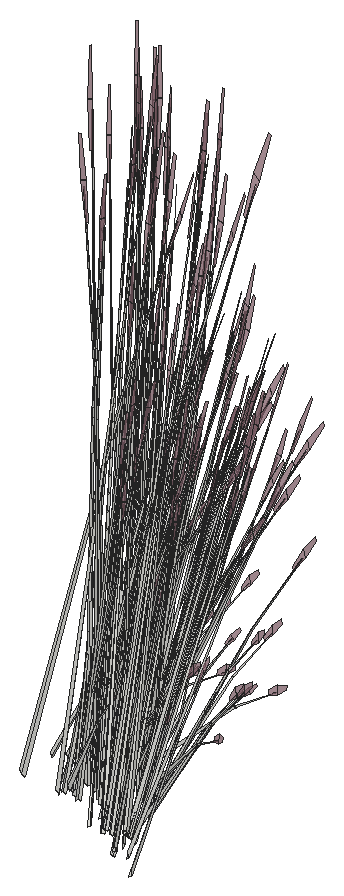
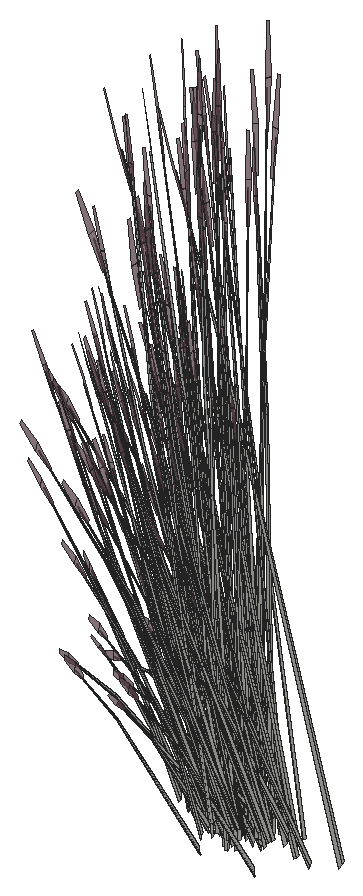
# SketchUp Ruby script. Lengths in inches.
U = 1.inch
M = Sketchup.active_model
def pt(a) = Geom::Point3d.new(a.map { |v| v * U })
def face(e, loops, mat)
  f = e.add_face(loops[0].map { |a| pt(a) })
  loops[1..].each { |l| e.add_face(l.map { |a| pt(a) }).erase! }
  f.material = f.back_material = mat if mat
  f
end
# faces: each face lists its corners as indices into pts; further lists are holes
def faces(e, pts, list, mat = nil) = list.each { |f| face(e, (f[0].is_a?(Array) ? f : [f]).map { |l| l.map { |i| pts[i] } }, mat) }
# xy, xz, yz: faces in a plane at the given z, y or x. An outline is a flat list of corners, or four numbers for a rectangle; further outlines are holes
def ring(l) = l.size == 4 ? [[l[0], l[1]], [l[2], l[1]], [l[2], l[3]], [l[0], l[3]]] : l.each_slice(2).to_a
def flat(e, list, mat, &to3) = list.each { |f| face(e, (f[0].is_a?(Array) ? f : [f]).map { |l| ring(l).map { |u, v| to3.(u, v) } }, mat) }
def xy(e, z, list, mat = nil) = flat(e, list, mat) { |x, y| [x, y, z] }
def xz(e, y, list, mat = nil) = flat(e, list, mat) { |x, z| [x, y, z] }
def yz(e, x, list, mat = nil) = flat(e, list, mat) { |y, z| [x, y, z] }
def lines(e, pts, list) = list.each { |a, b| e.add_line(pt(pts[a]), pt(pts[b])) }
# prism: a flat outline (further loops are holes) pulled along v
def prism(e, loops, v, mat = nil)
  f = face(e, loops, mat); d = Geom::Vector3d.new(v.map { |x| x * U })
  f.pushpull(f.normal.samedirection?(d) ? d.length : -d.length)
end
def box(e, o, s, mat = nil) = prism(e, [[o, [o[0] + s[0], o[1], o[2]], [o[0] + s[0], o[1] + s[1], o[2]], [o[0], o[1] + s[1], o[2]]]], [0, 0, s[2]], mat)
def at(x, y, z, deg = 0) = Geom::Transformation.translation(pt([x, y, z])) * Geom::Transformation.rotation(ORIGIN, Z_AXIS, deg.degrees)
def axes(o, x, y, z) = Geom::Transformation.new([*x, 0, *y, 0, *z, 0, *pt(o).to_a, 1])
def part(name) = M.definitions.add(name)
# library, detail: a bought-in or finely detailed component or shape, given as its bounding box
def library(name, o, s) = part(name).tap { |d| box(d.entities, o, s) }
def detail(e, o, s) = box(e.add_group.entities, o, s)
def put(e, d, t, mat = nil) = e.add_instance(d, t).tap { |i| i.material = mat if mat }
def group(e, t, mat = nil) = e.add_group.tap { |g| g.transformation = t; g.material = mat if mat }.entities
root = M.entities
M.materials.add("LightPink_Translucent").color = [144, 107, 117]
M.materials["LightPink_Translucent"].alpha = 0.75
c1 = part("blade")
p = [[2.15,0.21,22],[0,0.17,0],[0.09,0.45,0],[2.18,0.31,22],[2.29,0.31,22],[0.38,0.45,0],
  [2.48,0.24,33],[2.49,0.24,33],[2.48,0.22,33]]
faces(c1.entities,p,[[0,1,2,3],[4,5,2,3],[6,3,4,7],[8,0,3,6]])
c2 = part("seeds")
p = [[0.3,-0.1,1.38],[-0.01,-0.03,1.59],[-0.01,-0.03,0.03],[0.14,-0.07,-0.07],[0.29,-0.03,3],[0.15,0.01,3.11]]
faces(c2.entities,p,[[0,1,2,3],[1,0,4,5]],"LightPink_Translucent")
c3 = part("blade with seeds")
put(c3.entities,c1,at(0,0,0))
put(c3.entities,c2,axes([2.4,0.25,30.99],[1.5799,-0.05474,1.17369],[-0.12525,1.92788,0.29478],[-0.07173,-0.02425,1.56792]))
put(root,c3,axes([679.03,338.02,392.3],[-0.2167,0.29065,0.95334],[-0.18626,-0.3905,0.70045],[0.17898,-0.09785,0.20998]))
put(root,c3,axes([683.1,338.02,392.3],[-0.2167,0.29065,0.95334],[-0.18626,-0.3905,0.70045],[0.17898,-0.09785,0.20998]))
put(root,c3,axes([687.03,333.57,393.93],[-0.47939,0.19405,0.05337],[-0.23464,-0.35385,0.42015],[0.0463,0.15598,0.64067]))
put(root,c3,axes([685.74,333.11,393.76],[-0.4402,0.30062,-0.29394],[-0.41671,-0.34326,0.37948],[-0.0634,0.1744,0.72609]))
put(root,c3,axes([684.22,333.02,393.91],[-0.01617,0.11299,1.45204],[0.45894,0.39307,-0.22964],[-0.12015,0.18588,0.11645]))
put(root,c3,axes([685.69,332.76,394.48],[0.71502,0.02829,-0.11203],[-0.01954,0.53563,-0.62183],[-0.04967,0.20629,0.94486]))
put(root,c3,axes([687.01,333.36,394.18],[0.63664,-0.26583,-0.10093],[0.31286,0.47181,-0.56021],[0.084,0.19882,0.85122]))
put(root,c3,axes([687.2,333.53,394.2],[-0.64106,-0.14927,0.44225],[0.21921,-0.49074,0.36465],[0.03852,0.19299,0.91512]))
put(root,c3,axes([686.02,334.27,392.3],[-0.01684,-0.3395,0.95334],[0.42072,0.24214,0.70045],[-0.08274,0.16182,0.20998]))
put(root,c3,axes([678.72,339.11,393.76],[0.56631,-0.0816,-0.29394],[0.14954,0.46647,0.37948],[0.16229,-0.12529,0.72609]))
put(root,c3,axes([682.79,339.11,393.76],[0.56631,-0.0816,-0.29394],[0.14954,0.46647,0.37948],[0.16229,-0.12529,0.72609]))
put(root,c3,axes([687.13,333.46,391.24],[0.10529,-0.03107,1.46364],[0.63335,0.17101,-0.2236],[0.01852,0.19274,0.24931]))
put(root,c3,axes([679.47,339.53,392.21],[-0.07581,-0.65151,-0.24149],[0.7896,-0.03939,-0.41502],[0.13904,-0.08678,1.32557]))
put(root,c3,axes([686.18,332.96,394.15],[0.46573,0.38364,-0.47077],[-0.49199,0.33598,-0.36465],[-0.07086,0.19492,0.90078]))
put(root,c3,axes([682.33,339.38,394.19],[-0.56631,0.0816,0.29394],[-0.14954,-0.46647,-0.37948],[0.16229,-0.12529,0.72609]))
put(root,c3,axes([685.67,333.54,392.34],[0.59102,-0.10111,0.05401],[0.13587,0.40735,-0.71633],[-0.03747,0.2062,0.64209]))
put(root,c3,axes([687.56,333.34,393.89],[0.63954,0.14313,-0.42412],[-0.21921,0.49074,-0.32852],[0.05864,0.19758,0.81151]))
put(root,c3,axes([687.92,332.32,393.22],[-0.14872,-0.18332,1.42242],[0.6872,-0.15433,0.11501],[0.15531,0.28779,0.60807]))
put(root,c3,axes([679.36,338.09,391.68],[0.60696,0.14127,-0.25712],[-0.15283,0.49751,0.25712],[0.12236,-0.05737,1.15348]))
put(root,c3,axes([687.27,333.64,393.76],[-0.19614,0.43908,-0.29394],[-0.57222,-0.12807,0.37948],[0.05247,0.17678,0.72609]))
put(root,c3,axes([686.03,332.79,394.43],[-0.01693,0.52814,-0.65454],[-0.71285,-0.03547,0.07899],[-0.07523,0.22375,0.92591]))
put(root,c3,axes([684.17,334.18,393.91],[0.07381,-0.03447,1.47228],[0.61004,0.22929,-0.13912],[-0.01434,0.19091,0.26054]))
put(root,c3,axes([678.77,339.31,393.93],[0.44663,0.24013,0.05337],[-0.26003,0.34195,0.42015],[0.14319,-0.11055,0.64067]))
put(root,c3,axes([682.84,339.31,393.93],[0.44663,0.24013,0.05337],[-0.26003,0.34195,0.42015],[0.14319,-0.11055,0.64067]))
put(root,c3,axes([678.65,339.21,393.93],[0.16135,0.52549,0.39842],[-0.63294,0.0912,0.32852],[0.18654,-0.12359,0.82444]))
put(root,c3,axes([682.72,339.21,393.93],[0.16135,0.52549,0.39842],[-0.63294,0.0912,0.32852],[0.18654,-0.12359,0.82444]))
put(root,c3,axes([680.36,339.84,393.91],[0.09028,-0.08697,1.45204],[-0.11555,-0.53348,-0.22964],[0.22652,-0.10115,0.11645]))
put(root,c3,axes([684.42,339.84,393.91],[0.09028,-0.08697,1.45204],[-0.11555,-0.53348,-0.22964],[0.22652,-0.10115,0.11645]))
put(root,c3,axes([686.71,332.41,393.22],[-0.01592,-0.21915,1.42242],[0.69015,0.14538,0.11501],[-0.04269,0.3123,0.60807]))
put(root,c3,axes([687.33,333.24,394.13],[0.31051,0.46426,-0.58968],[-0.63919,0.25873,0.07116],[0.07261,0.22432,0.83415]))
put(root,c3,axes([685.53,333.97,392.15],[0.2053,-0.09007,1.18691],[0.50689,0.27159,-0.25526],[-0.15087,0.235,0.50747]))
put(root,c3,axes([679.57,340.04,392.02],[0.73304,0.27674,0.19974],[-0.35279,0.57501,0.41502],[0,-0.13255,1.3325]))
put(root,c3,axes([686.86,334.41,393.91],[0.08247,0.09194,1.45204],[0.66552,0.03612,-0.22964],[0.06692,0.20277,0.11645]))
put(root,c3,axes([679.33,339.66,392.26],[-0.70648,0.03525,0.37133],[-0.06389,-0.58508,-0.17871],[0.12647,-0.0593,1.19224]))
put(root,c3,axes([678.58,340.65,394.18],[-0.32734,-0.51701,-0.10093],[0.58097,-0.25407,-0.56021],[0.24483,-0.06821,0.85122]))
put(root,c3,axes([682.65,340.65,394.18],[-0.32734,-0.51701,-0.10093],[0.58097,-0.25407,-0.56021],[0.24483,-0.06821,0.85122]))
put(root,c3,axes([678.55,340.21,393.89],[0.17625,-0.51936,-0.42412],[0.60429,0.17802,-0.32852],[0.2433,-0.04762,0.81151]))
put(root,c3,axes([682.62,340.21,393.89],[0.17625,-0.51936,-0.42412],[0.60429,0.17802,-0.32852],[0.2433,-0.04762,0.81151]))
put(root,c3,axes([677.59,338.1,391.97],[0.40676,-0.57214,0],[0.68052,0.31907,-0.42834],[0.15499,0.07267,1.3588]))
put(root,c3,axes([681.66,338.1,391.97],[0.40676,-0.57214,0],[0.68052,0.31907,-0.42834],[0.15499,0.07267,1.3588]))
put(root,c3,axes([685.79,333.53,392.79],[0.01429,-0.29475,1.28107],[0.64291,0.15569,0.17703],[-0.0557,0.31414,0.60492]))
put(root,c3,axes([679.19,340.36,391.65],[-0.41902,0.06852,1.17514],[-0.0667,-0.54541,0.06726],[0.29348,-0.08255,0.6687]))
put(root,c3,axes([683.26,340.36,391.65],[-0.41902,0.06852,1.17514],[-0.0667,-0.54541,0.06726],[0.29348,-0.08255,0.6687]))
put(root,c3,axes([679.96,339.875,391.875],[-0.40335,-0.3651,-0.05385],[0.44175,-0.33453,-0.24415],[0.12517,-0.02355,0.8053]))
put(root,c3,axes([684.03,339.875,391.875],[-0.40335,-0.3651,-0.05385],[0.44175,-0.33453,-0.24415],[0.12517,-0.02355,0.8053]))
put(root,c3,axes([680.33,339.92,391.83],[0,-0.66065,0],[0.81352,0,0],[0,0,1.48949]))
put(root,c3,axes([681.3125,338.39,392.06],[-0.60889,-0.28548,0.4121],[0.36394,-0.51192,0],[0.13868,0.06502,1.30728]))
put(root,c3,axes([678.43,340.4,394.13],[0.57168,-0.25217,-0.58968],[0.3186,0.51908,0.07116],[0.27622,-0.05897,0.83415]))
put(root,c3,axes([682.5,340.4,394.13],[0.57168,-0.25217,-0.58968],[0.3186,0.51908,0.07116],[0.27622,-0.05897,0.83415]))
put(root,c3,axes([679.94,339.51,391.96],[-0.53943,0.51816,0.37976],[-0.64086,-0.4574,0.14902],[0.13005,-0.05171,1.31851]))
put(root,c3,axes([679,338.65,392.05],[-0.18794,0.56744,0.14643],[-0.68774,-0.16058,0.29122],[0.1188,-0.00276,1.33138]))
put(root,c3,axes([678.35,340.5,394.19],[-0.54068,-0.15928,0.29394],[0.1577,-0.46469,-0.37948],[0.21769,-0.04261,0.72609]))
put(root,c3,axes([682.42,340.5,394.19],[-0.54068,-0.15928,0.29394],[0.1577,-0.46469,-0.37948],[0.21769,-0.04261,0.72609]))
put(root,c3,axes([674.65,339.11,391.32],[-0.64037,0.22859,1.07011],[-0.20382,-0.65589,0.4158],[0.39323,0.01091,1.21713]))
put(root,c3,axes([678.72,339.11,391.32],[-0.64037,0.22859,1.07011],[-0.20382,-0.65589,0.4158],[0.39323,0.01091,1.21713]))
put(root,c3,axes([680.44,339.28,392.17],[0.12551,-0.50956,0.12018],[0.6132,0.08845,-0.34318],[0.1116,0.05232,1.05198]))
put(root,c3,axes([679.65,340,391.24],[-0.034,-0.08668,1.46364],[0.23582,-0.50706,-0.2236],[0.23788,-0.00729,0.24931]))
put(root,c3,axes([683.72,340,391.24],[-0.034,-0.08668,1.46364],[0.23582,-0.50706,-0.2236],[0.23788,-0.00729,0.24931]))
put(root,c3,axes([680.18,339.42,392.26],[-0.39083,-0.47924,0.37133],[0.59199,-0.33747,-0.17871],[0.12647,0.0593,1.19224]))
put(root,c3,axes([680.38,339.45,392.21],[0.65687,-0.37907,-0.24149],[0.43681,0.53562,-0.41502],[0.16207,0.0544,1.32557]))
put(root,c3,axes([678.92,340.45,393.76],[0.54068,0.15928,-0.29394],[-0.1577,0.46469,0.37948],[0.21769,-0.04261,0.72609]))
put(root,c3,axes([682.99,340.45,393.76],[0.54068,0.15928,-0.29394],[-0.1577,0.46469,0.37948],[0.21769,-0.04261,0.72609]))
put(root,c3,axes([677.96,338.44,391.67],[0.60889,0.28548,-0.4121],[-0.36394,0.51192,0],[0.13868,0.06502,1.30728]))
put(root,c3,axes([682.03,338.44,391.67],[0.60889,0.28548,-0.4121],[-0.36394,0.51192,0],[0.13868,0.06502,1.30728]))
put(root,c3,axes([680.88,340.07,391.83],[0.72788,0,0],[0,0.59111,0],[0,0,1.48078]))
put(root,c3,axes([681.08,338.68,392.05],[-0.6991,0.15154,0.14643],[-0.17263,-0.56398,0.29122],[0.06235,0.08217,1.33138]))
put(root,c3,axes([677.45,339.87,393.22],[-0.26985,0.01293,1.42242],[0.17902,-0.56047,0.11501],[0.38456,0.03467,0.60807]))
put(root,c3,axes([681.52,339.87,393.22],[-0.26985,0.01293,1.42242],[0.17902,-0.56047,0.11501],[0.38456,0.03467,0.60807]))
put(root,c3,axes([681.86,338.65,391.68],[0.15283,0.49751,-0.25712],[-0.60696,0.14127,0.25712],[0.12236,0.05737,1.15348]))
put(root,c3,axes([678.84,340.64,393.93],[0.23895,0.38931,0.05337],[-0.43573,0.19055,0.42015],[0.19208,-0.0376,0.64067]))
put(root,c3,axes([682.91,340.64,393.93],[0.23895,0.38931,0.05337],[-0.43573,0.19055,0.42015],[0.19208,-0.0376,0.64067]))
put(root,c3,axes([680.64,339.77,391.98],[-0.82229,-0.1203,0.40835],[0.16734,-0.67942,0.16024],[0.12017,0.06561,1.41775]))
put(root,c3,axes([678.79,340.51,393.93],[-0.18381,0.5206,0.39842],[-0.60429,-0.17802,0.32852],[0.23764,-0.03129,0.82444]))
put(root,c3,axes([682.86,340.51,393.93],[-0.18381,0.5206,0.39842],[-0.60429,-0.17802,0.32852],[0.23764,-0.03129,0.82444]))
put(root,c3,axes([680.78,341.375,391.8125],[0.68303,-0.19373,-0.15934],[0.24001,0.55805,0.00007],[0.07539,-0.02141,1.44335]))
put(root,c3,axes([680.86,340.32,391.84],[0.45414,0.3688,0],[-0.45414,0.3688,0],[0,0,1.40491]))
put(root,c3,axes([682.09,340.16,392.05],[-0.51116,-0.4159,0.14643],[0.51512,-0.4034,0.29122],[-0.05645,0.08494,1.33138]))
put(root,c3,axes([677.08,339.53,391.71],[0.67676,0.09361,-0.51753],[-0.14281,0.57742,-0.13583],[0.20196,0.06997,1.14236]))
put(root,c3,axes([681.15,339.53,391.71],[0.67676,0.09361,-0.51753],[-0.14281,0.57742,-0.13583],[0.20196,0.06997,1.14236]))
put(root,c3,axes([680.07,340.54,392.3],[-0.40197,0.09426,0.95334],[0.18921,-0.38956,0.70045],[0.21325,0.02666,0.20998]))
put(root,c3,axes([684.14,340.54,392.3],[-0.40197,0.09426,0.95334],[0.18921,-0.38956,0.70045],[0.21325,0.02666,0.20998]))
put(root,c3,axes([680.86,339.89,392.26],[0.31565,-0.51449,0.37133],[0.65588,0.24761,-0.17871],[0,0.1186,1.19224]))
put(root,c3,axes([679.88,342.19,393.91],[-0.05883,-0.04999,1.47228],[0.12868,-0.53581,-0.13912],[0.23172,-0.03423,0.26054]))
put(root,c3,axes([683.95,342.19,393.91],[-0.05883,-0.04999,1.47228],[0.12868,-0.53581,-0.13912],[0.23172,-0.03423,0.26054]))
put(root,c3,axes([680.73,340.19,391.9],[0,0.66033,-0.04679],[-0.81352,0,0],[0,0.02075,1.48875]))
put(root,c3,axes([680.79,339.72,391.83],[0.39083,0.47924,-0.37133],[-0.59199,0.33747,0.17871],[0.12647,0.0593,1.19224]))
put(root,c3,axes([679.37,341.74,393.26],[-0.12452,-0.47997,-0.02898],[0.58854,-0.11034,-0.1314],[0.1229,0.03043,0.43341]))
put(root,c3,axes([683.4375,341.74,393.26],[-0.12452,-0.47997,-0.02898],[0.58854,-0.11034,-0.1314],[0.1229,0.03043,0.43341]))
put(root,c3,axes([677.84,341.73,394.18],[0.03484,-0.58066,-0.10093],[0.65957,0.01587,-0.56021],[0.25402,0.04034,0.85122]))
put(root,c3,axes([681.91,341.73,394.18],[0.03484,-0.58066,-0.10093],[0.65957,0.01587,-0.56021],[0.25402,0.04034,0.85122]))
put(root,c3,axes([682.51,340.18,392.06],[0,-0.57097,0.4121],[0.72788,0,0],[0,0.13004,1.30728]))
put(root,c3,axes([681.13,340.01,392.17],[0.60616,-0.16651,0.12018],[0.21227,0.47548,-0.34318],[0,0.10465,1.05198]))
put(root,c3,axes([677.74,341.5,394.19],[-0.37017,-0.35748,0.29394],[0.42268,-0.3384,-0.37948],[0.21476,0.05149,0.72609]))
put(root,c3,axes([681.81,341.5,394.19],[-0.37017,-0.35748,0.29394],[0.42268,-0.3384,-0.37948],[0.21476,0.05149,0.72609]))
put(root,c3,axes([675.13,341.17,392.15],[-0.15668,-0.14043,1.18691],[0.20386,-0.46454,-0.25526],[0.31701,0.06293,0.50747]))
put(root,c3,axes([679.3125,341.17,392.15],[-0.15668,-0.14043,1.18691],[0.20386,-0.46454,-0.25526],[0.31701,0.06293,0.50747]))
put(root,c3,axes([683.38,341.17,392.15],[-0.15668,-0.14043,1.18691],[0.20386,-0.46454,-0.25526],[0.31701,0.06293,0.50747]))
put(root,c3,axes([680.58,341.68,391.83],[0.65588,0.25634,0],[-0.31565,0.53263,0],[0,0,1.45212]))
put(root,c3,axes([678.42,341.38,393.91],[0.13956,-0.00966,1.45204],[0.38281,-0.44358,-0.22964],[0.24825,0.05855,0.11645]))
put(root,c3,axes([682.48,341.38,393.91],[0.13956,-0.00966,1.45204],[0.38281,-0.44358,-0.22964],[0.24825,0.05855,0.11645]))
put(root,c3,axes([677.875,341.45,394.13],[0.65035,0.01375,-0.58968],[-0.04368,0.5789,0.07116],[0.27552,0.06109,0.83415]))
put(root,c3,axes([681.94,341.45,394.13],[0.65035,0.01375,-0.58968],[-0.04368,0.5789,0.07116],[0.27552,0.06109,0.83415]))
put(root,c3,axes([680.35,341.46,391.9],[0.28286,0.65594,-0.0499],[-0.80821,0.22985,0],[0.00988,0.02291,1.42904]))
put(root,c3,axes([683.01,340.28,391.97],[0.81352,0,0],[0,0.63814,-0.42834],[0,0.14534,1.3588]))
put(root,c3,axes([682.68,340.6,391.83],[-0.81312,-0.00457,-0.0413],[0,-0.63814,0.41452],[-0.02555,0.14527,1.31432]))
put(root,c3,axes([680.92,340.05,392.21],[0.73268,0.27244,-0.24149],[-0.35279,0.57501,-0.41502],[0.02303,0.14118,1.32557]))
put(root,c3,axes([678.27,341.6875,393.76],[0.37017,0.35748,-0.29394],[-0.42268,0.3384,0.37948],[0.21476,0.05149,0.72609]))
put(root,c3,axes([682.33,341.6875,393.76],[0.37017,0.35748,-0.29394],[-0.42268,0.3384,0.37948],[0.21476,0.05149,0.72609]))
put(root,c3,axes([682.51,340.7,391.68],[-0.45414,0.35624,-0.25712],[-0.45414,-0.35624,0.25712],[0,0.11474,1.15348]))
put(root,c3,axes([678.08,341.83,393.93],[-0.03276,0.43418,0.05337],[-0.49468,-0.0119,0.42015],[0.18949,0.04543,0.64067]))
put(root,c3,axes([682.15,341.83,393.93],[-0.03276,0.43418,0.05337],[-0.49468,-0.0119,0.42015],[0.18949,0.04543,0.64067]))
put(root,c3,axes([678.12,341.6875,393.93],[-0.47971,0.37622,0.39842],[-0.41372,-0.39954,0.32852],[0.22506,0.0694,0.82444]))
put(root,c3,axes([682.19,341.6875,393.93],[-0.47971,0.37622,0.39842],[-0.41372,-0.39954,0.32852],[0.22506,0.0694,0.82444]))
put(root,c3,axes([680.67,342.12,394.19],[-0.10048,-0.4599,0.29394],[0.5744,-0.12144,-0.37948],[0.15428,0.13179,0.72609]))
put(root,c3,axes([682.82,340.71,391.67],[0,0.57097,-0.4121],[-0.72788,0,0],[0,0.13004,1.30728]))
put(root,c3,axes([676.9375,340.77,393.22],[-0.24166,-0.09837,1.42242],[0.50011,-0.41269,0.11501],[0.3117,0.18617,0.60807]))
put(root,c3,axes([681.01,340.77,393.22],[-0.24166,-0.09837,1.42242],[0.50011,-0.41269,0.11501],[0.3117,0.18617,0.60807]))
put(root,c3,axes([681.05,339.48,393.71],[-0.56218,-0.29666,1.14775],[0.59361,-0.46189,0.49522],[0.18138,0.27836,1.10941]))
put(root,c3,axes([681.9,341.89,392.3],[-0.36631,-0.16417,0.95334],[0.47299,-0.16681,0.70045],[0.12758,0.1413,0.20998]))
put(root,c3,axes([676.54,342.36,394.18],[0.38768,-0.48872,-0.10093],[0.56143,0.28156,-0.56021],[0.19516,0.13808,0.85122]))
put(root,c3,axes([680.61,342.36,394.18],[0.38768,-0.48872,-0.10093],[0.56143,0.28156,-0.56021],[0.19516,0.13808,0.85122]))
put(root,c3,axes([680.11,342.77,393.91],[0.00193,-0.06913,1.47228],[0.55753,-0.30498,-0.13912],[0.19366,0.10886,0.26054]))
put(root,c3,axes([677.93,342.5,391.24],[0.0474,-0.08243,1.46364],[0.59674,-0.24277,-0.2236],[0.18092,0.12565,0.24931]))
put(root,c3,axes([682,342.5,391.24],[0.0474,-0.08243,1.46364],[0.59674,-0.24277,-0.2236],[0.18092,0.12565,0.24931]))
put(root,c3,axes([681.21,340.63,391.74],[0.23855,0.52277,-0.57446],[-0.68718,0.18827,-0.15077],[0.02637,0.17702,1.26801]))
put(root,c3,axes([677,342.12,393.89],[0.64198,-0.13573,-0.42412],[0.1123,0.514,-0.32852],[0.17243,0.1473,0.81151]))
put(root,c3,axes([681.07,342.12,393.89],[0.64198,-0.13573,-0.42412],[0.1123,0.514,-0.32852],[0.17243,0.1473,0.81151]))
put(root,c3,axes([679.29,342.2,394.19],[0.19614,-0.43908,0.29394],[0.57222,0.12807,-0.37948],[0.05247,0.17678,0.72609]))
put(root,c3,axes([681.96,342.64,392.21],[-0.4172,-0.01791,0.872],[0.27552,-0.38032,0.48145],[0.16481,0.13512,0.68401]))
put(root,c3,axes([680.76,342.54,393.93],[-0.29569,0.36271,0.05337],[-0.42107,-0.21117,0.42015],[0.13613,0.11629,0.64067]))
put(root,c3,axes([680.0625,343.76,394.6875],[0.44958,-0.32756,-0.05385],[0.41194,0.35875,-0.24415],[0.029,0.10165,0.8053]))
put(root,c3,axes([680.88,342.4375,393.93],[-0.64708,0.13103,0.39842],[-0.1123,-0.514,0.32852],[0.15218,0.15149,0.82444]))
put(root,c3,axes([680.6,341.72,392.15],[0.01148,-0.18927,1.18691],[0.54864,-0.21141,-0.25526],[0.16937,0.22654,0.50747]))
put(root,c3,axes([679.1,342.38,394.18],[0.63664,-0.26583,-0.10093],[0.31286,0.47181,-0.56021],[0.084,0.19882,0.85122]))
put(root,c3,axes([679.65,342.36,393.89],[0.63954,0.14313,-0.42412],[-0.21921,0.49074,-0.32852],[0.05864,0.19758,0.81151]))
put(root,c3,axes([680.01,341.34,393.22],[-0.14872,-0.18332,1.42242],[0.6872,-0.15433,0.11501],[0.15531,0.28779,0.60807]))
put(root,c3,axes([679.41,342.26,394.13],[0.31051,0.46426,-0.58968],[-0.63919,0.25873,0.07116],[0.07261,0.22432,0.83415]))
